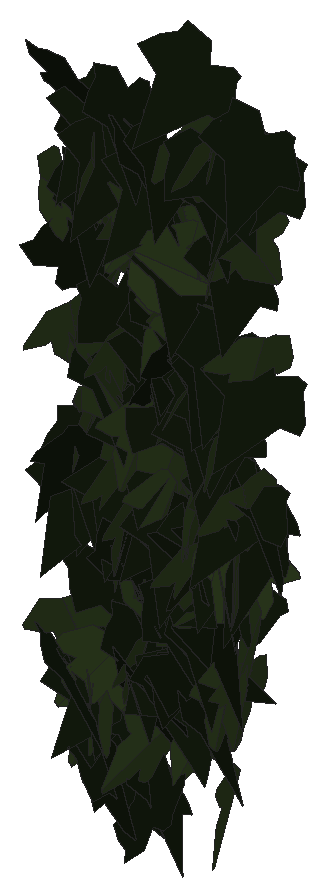
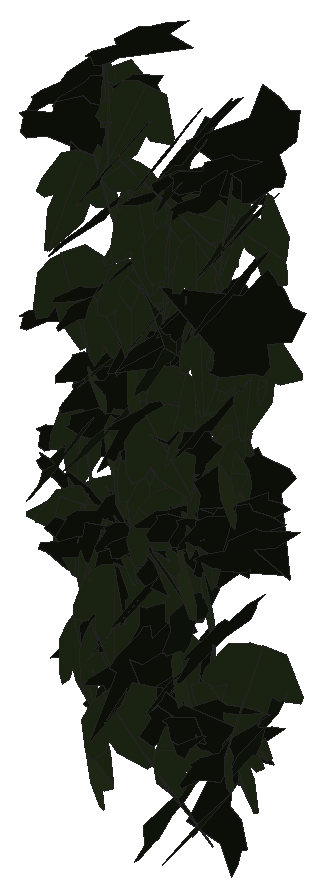
# SketchUp Ruby script. Lengths in inches.
U = 1.inch
M = Sketchup.active_model
def pt(a) = Geom::Point3d.new(a.map { |v| v * U })
def face(e, loops, mat)
  f = e.add_face(loops[0].map { |a| pt(a) })
  loops[1..].each { |l| e.add_face(l.map { |a| pt(a) }).erase! }
  f.material = f.back_material = mat if mat
  f
end
# faces: each face lists its corners as indices into pts; further lists are holes
def faces(e, pts, list, mat = nil) = list.each { |f| face(e, (f[0].is_a?(Array) ? f : [f]).map { |l| l.map { |i| pts[i] } }, mat) }
# xy, xz, yz: faces in a plane at the given z, y or x. An outline is a flat list of corners, or four numbers for a rectangle; further outlines are holes
def ring(l) = l.size == 4 ? [[l[0], l[1]], [l[2], l[1]], [l[2], l[3]], [l[0], l[3]]] : l.each_slice(2).to_a
def flat(e, list, mat, &to3) = list.each { |f| face(e, (f[0].is_a?(Array) ? f : [f]).map { |l| ring(l).map { |u, v| to3.(u, v) } }, mat) }
def xy(e, z, list, mat = nil) = flat(e, list, mat) { |x, y| [x, y, z] }
def xz(e, y, list, mat = nil) = flat(e, list, mat) { |x, z| [x, y, z] }
def yz(e, x, list, mat = nil) = flat(e, list, mat) { |y, z| [x, y, z] }
def lines(e, pts, list) = list.each { |a, b| e.add_line(pt(pts[a]), pt(pts[b])) }
# prism: a flat outline (further loops are holes) pulled along v
def prism(e, loops, v, mat = nil)
  f = face(e, loops, mat); d = Geom::Vector3d.new(v.map { |x| x * U })
  f.pushpull(f.normal.samedirection?(d) ? d.length : -d.length)
end
def box(e, o, s, mat = nil) = prism(e, [[o, [o[0] + s[0], o[1], o[2]], [o[0] + s[0], o[1] + s[1], o[2]], [o[0], o[1] + s[1], o[2]]]], [0, 0, s[2]], mat)
def at(x, y, z, deg = 0) = Geom::Transformation.translation(pt([x, y, z])) * Geom::Transformation.rotation(ORIGIN, Z_AXIS, deg.degrees)
def axes(o, x, y, z) = Geom::Transformation.new([*x, 0, *y, 0, *z, 0, *pt(o).to_a, 1])
def part(name) = M.definitions.add(name)
# library, detail: a bought-in or finely detailed component or shape, given as its bounding box
def library(name, o, s) = part(name).tap { |d| box(d.entities, o, s) }
def detail(e, o, s) = box(e.add_group.entities, o, s)
def put(e, d, t, mat = nil) = e.add_instance(d, t).tap { |i| i.material = mat if mat }
def group(e, t, mat = nil) = e.add_group.tap { |g| g.transformation = t; g.material = mat if mat }.entities
root = M.entities
M.materials.add("efeu1").color = [18, 25, 13]
M.materials.add("efeu2").color = [43, 57, 29]
c1 = part("ivyleaf_9")
p = [[1.54,2.16,1.25],[1.36,2.04,1.19],[-0.21,0.99,0.68],[-0.71,1.11,0.82],[-0.85,0.86,0.67],[-0.8,0.17,0.21],
  [-0.9,-0.01,0.1],[-0.67,-0.16,-0.02],[-0.08,-0.08,-0.05],[-0.03,-0.6,-0.4],[0.65,-0.88,-0.66],[0.83,-0.6,-0.49],
  [1.29,-0.42,-0.43],[1.8125,-0.07,-0.26],[1.21,0.44,0.15]]
faces(c1.entities,p,[[0,1,2,3,4,5,6,7,8,9,10,11,12,13,14]],"efeu1")
c2 = part("ivyleaf_10")
p = [[0,0.5,-0.03],[-0.0625,2.02,-0.43],[-0.19,2.01,-0.46],[-0.54,1.05,-0.29],[-0.52,0.625,-0.18],[-0.83,0.76,-0.28],
  [-1.16,0.64,-0.33],[-1.15,0.33,-0.24],[-0.77,-0.39,0.02],[-0.3,-0.51,0.16],[0.04,-0.48,0.23],[-0.02,2.01,-0.4375],
  [-0.06,2.01,-0.43],[0.04,-0.49,0.23],[0.67,-0.49,0.14],[1.38,0.36,-0.2],[1.375,0.51,-0.24],[0.81,0.65,-0.19],
  [0.62,0.59,-0.15],[0.6,1.09,-0.28],[0.5,1.23,-0.31]]
faces(c2.entities,p,[[0,1,2,3,4,5,6,7,8,9,10],[11,12,0,13,14,15,16,17,18,19,20]],"efeu2")
put(root,c1,axes([22.86,222.96,230.22],[0.08833,-0.4463,-0.20739],[-0.02573,0.20623,-0.45476],[0.49146,0.09101,0.01347]))
put(root,c2,axes([23.15,223.3,223.84],[-0.02881,-0.15896,0.47318],[0.07947,-0.46938,-0.15285],[0.4928,0.0664,0.05231]))
put(root,c2,axes([23.02,223.03,227.23],[0.1477,-0.47388,0.06016],[0.02404,-0.05552,-0.49633],[0.47708,0.14951,0.00638]))
put(root,c2,axes([21.75,222.98,231.33],[-0.01778,-0.00473,0.49966],[0.49964,-0.00651,0.01771],[0.00633,0.49994,0.00496]))
put(root,c1,axes([22.25,223.23,231.43],[0.03847,-0.47216,0.15996],[0.03093,-0.15786,-0.47342],[0.49756,0.04632,0.01706]))
put(root,c2,axes([22.98,222.91,229.69],[-0.00486,-0.49041,-0.09735],[0.00651,0.09728,-0.4904],[0.49993,-0.00603,0.00544]))
put(root,c1,axes([23.97,223.3125,233.67],[-0.30955,-0.34814,0.18161],[-0.04977,-0.1946,-0.45788],[0.38949,-0.30155,0.08582]))
put(root,c2,axes([24.42,223.2,228.96],[0.19071,-0.36763,0.28013],[0.1358,-0.2451,-0.41411],[0.4418,0.23404,0.00636]))
put(root,c2,axes([24.61,223.16,227.08],[-0.16491,0.29275,-0.37027],[0.10502,-0.35963,-0.33112],[-0.46019,-0.18698,0.05713]))
put(root,c1,axes([24.34,223.07,226.03],[-0.15159,-0.00545,-0.47643],[0.47475,0.04065,-0.15152],[0.04038,-0.49832,-0.00715]))
put(root,c2,axes([24.29,222.95,232.79],[0.04442,-0.49195,-0.07754],[0.00767,0.07852,-0.49374],[0.49796,0.04267,0.01452]))
put(root,c1,axes([24.39,223.27,229.91],[-0.11221,-0.47814,0.09379],[-0.00603,-0.09487,-0.49088],[0.48721,-0.11129,0.01552]))
put(root,c2,axes([24.09,223,226.91],[-0.07675,-0.49389,-0.01342],[0.00355,0.01303,-0.49982],[0.49406,-0.07682,0.00151]))
put(root,c1,axes([23.09,222.97,226.24],[-0.12939,-0.06336,0.47879],[0.45684,-0.1769,0.10004],[0.15672,0.46335,0.10367]))
put(root,c1,axes([25.01,223.3125,229.57],[-0.27863,-0.39715,0.12099],[-0.01077,-0.13875,-0.48024],[0.41503,-0.27022,0.06877]))
put(root,c1,axes([23.63,223.29,230.82],[-0.02142,-0.47188,0.16393],[0.03554,-0.16511,-0.47061],[0.49828,-0.00851,0.04061]))
put(root,c2,axes([22.625,222.99,231.35],[-0.32203,0.11672,-0.36424],[0.34419,-0.11924,-0.34251],[-0.16681,-0.47134,-0.00355]))
put(root,c1,axes([22.29,223.03,227.92],[-0.03278,0.36396,-0.34126],[0.02608,-0.34028,-0.36542],[-0.49824,-0.04176,0.00332]))
put(root,c2,axes([23.7,223.25,230.22],[-0.13326,-0.35698,0.32374],[-0.00762,-0.33429,-0.37174],[0.48185,-0.10401,0.08366]))
put(root,c1,axes([21.8,223.17,224.61],[0.2499,-0.3976,0.17165],[0.09149,-0.14523,-0.46961],[0.4233,0.26612,0.00017]))
put(root,c1,axes([23.68,222.56,229.48],[0.11001,0.28622,0.39494],[0.15441,0.3636,-0.30652],[-0.46266,0.18941,-0.0084]))
put(root,c2,axes([22.6875,222.92,228.73],[-0.29006,0.11419,-0.39093],[-0.36407,0.1424,0.31172],[0.18253,0.46549,0.00054]))
put(root,c1,axes([24.75,223.28,227.92],[-0.35549,-0.34847,0.04682],[-0.01764,-0.04882,-0.4973],[0.35116,-0.35522,0.02242]))
put(root,c2,axes([22.44,223.01,224.18],[0.43207,-0.21733,-0.12681],[-0.10618,0.07096,-0.48341],[0.22812,0.44467,0.01517]))
put(root,c2,axes([23.16,223.1875,228.45],[-0.14924,-0.43249,0.2017],[0.01101,-0.2144,-0.45157],[0.47708,-0.13035,0.07352]))
put(root,c2,axes([24.14,223.19,227.875],[0.20825,-0.41714,0.18063],[0.07426,-0.1648,-0.46618],[0.44846,0.22099,-0.00668]))
put(root,c2,axes([24.43,223.08,231.59],[0.27301,-0.41888,0.00251],[-0.00001,-0.003,-0.49999],[0.41889,0.27301,-0.00165]))
put(root,c2,axes([23.625,222.7,231.05],[0.09534,0.23118,0.43298],[0.17159,0.39754,-0.25004],[-0.45986,0.19626,-0.00353]))
put(root,c1,axes([23.35,223.37,231.8125],[-0.27472,-0.37614,0.18179],[-0.05475,-0.18328,-0.46196],[0.41416,-0.27373,0.05952]))
put(root,c1,axes([23.34,223.36,232.21],[0.01894,-0.43265,0.24992],[0.02312,-0.24907,-0.43293],[0.49911,0.02795,0.01057]))
put(root,c2,axes([22.1,222.96,229.67],[-0.17284,-0.45383,-0.11903],[0.05122,0.10784,-0.48554],[0.46637,-0.18004,0.00922]))
put(root,c1,axes([22.61,223.37,232.02],[-0.20321,-0.426,0.165],[-0.04127,-0.16273,-0.47097],[0.45497,-0.20504,0.03097]))
put(root,c1,axes([24.31,223.03,232.8],[-0.04489,-0.38512,-0.3157],[0.06678,0.30946,-0.38701],[0.49348,-0.07691,0.02365]))
put(root,c1,axes([23.59,223.14,226.02],[0.18729,-0.45597,-0.08375],[-0.0255,0.08006,-0.49289],[0.4629,0.1889,0.00673]))
put(root,c1,axes([23.85,222.79,225.46],[0.02851,0.00436,-0.49917],[0.1502,0.47674,0.01274],[0.47605,-0.15068,0.02587]))
put(root,c2,axes([22.46,222.91,231.89],[0.1637,-0.40747,-0.2391],[0.02953,0.26137,-0.42522],[0.47152,0.1251,0.10964]))
put(root,c1,axes([23.23,223.22,224.1],[0.37413,-0.24537,0.22321],[-0.18632,0.12292,0.44741],[-0.27444,-0.41795,0.00055]))
put(root,c1,axes([24.09,223.46,229.13],[-0.12274,-0.37882,0.30237],[0.08857,-0.32419,-0.37021],[0.47654,-0.03732,0.14668]))
put(root,c2,axes([24.92,223.18,230],[-0.19279,-0.45191,0.09277],[-0.01999,-0.09227,-0.49101],[0.4609,-0.19303,0.01751]))
put(root,c2,axes([24.78,223.03,227.96],[-0.12237,-0.46835,-0.12521],[0.04271,0.11822,-0.48394],[0.48291,-0.12914,0.01107]))
put(root,c1,axes([24.79,223.42,232.89],[-0.14424,-0.46381,0.11865],[-0.00796,-0.12157,-0.48493],[0.47868,-0.14178,0.02769]))
put(root,c2,axes([23.84,223.4,227.64],[0.0936,-0.27919,0.40409],[0.24151,-0.33204,-0.28535],[0.42768,0.2486,0.0727]))
put(root,c1,axes([23.18,223.43,229.44],[0.0297,-0.38591,0.31652],[0.10535,-0.30509,-0.38186],[0.48787,0.08938,0.06319]))
put(root,c2,axes([22.5,223.14,224.82],[0.41456,-0.01294,-0.27923],[-0.27895,0.01299,-0.41475],[0.01799,0.49966,0.00355]))
put(root,c1,axes([22.93,223.23,232.32],[0.27368,-0.41416,0.05971],[0.02588,-0.05446,-0.49635],[0.41765,0.27478,-0.00837]))
put(root,c1,axes([21.65,223.13,232.85],[0.34092,-0.17815,0.31943],[0.28597,-0.14241,-0.38463],[0.22803,0.44495,0.00479]))
put(root,c1,axes([23.5,222.83,222.9375],[-0.41726,0.18998,-0.19952],[-0.18595,0.07297,0.45836],[0.20328,0.45671,0.00975]))
put(root,c1,axes([22.14,223.43,227.125],[-0.27659,-0.40638,0.09142],[-0.02251,-0.09499,-0.49038],[0.41592,-0.27538,0.03425]))
put(root,c2,axes([22.98,223.17,226.13],[0.12027,-0.08451,-0.4779],[0.45878,-0.14078,0.14035],[-0.15828,-0.47227,0.04368]))
put(root,c1,axes([24.4,223.45,231],[-0.06149,-0.46571,0.17127],[0.05266,-0.17773,-0.46437],[0.4934,-0.03907,0.0709]))
put(root,c2,axes([24.32,223.32,225.09],[0.01246,-0.44884,0.21997],[0.1506,-0.20644,-0.42977],[0.47662,0.07696,0.13005]))
put(root,c1,axes([24.18,223.33,228.78],[-0.17737,-0.46356,-0.06046],[0.00638,0.06226,-0.49607],[0.46744,-0.17675,-0.01617]))
put(root,c1,axes([22.6875,223.35,232.84],[0.08267,-0.49019,0.05362],[0.00269,-0.05392,-0.49708],[0.49311,0.08248,-0.00628]))
put(root,c2,axes([22.02,223.06,225.36],[-0.43186,-0.22409,-0.11524],[0.10209,0.05347,-0.48654],[0.23038,-0.44376,-0.00043]))
put(root,c1,axes([23.86,223.42,225.55],[0.09728,-0.45755,0.17658],[0.04698,-0.1705,-0.46768],[0.48819,0.10758,0.00982]))
put(root,c1,axes([22.28,223.26,223.33],[-0.0292,-0.02934,-0.49828],[0.49591,0.05501,-0.0323],[0.05672,-0.4961,0.02589]))
put(root,c2,axes([23.41,223.34,227.47],[-0.08875,-0.45001,0.19903],[0.02537,-0.20616,-0.45481],[0.49141,-0.07063,0.05943]))
put(root,c1,axes([22.71,223.42,225.95],[0.13874,-0.29865,0.37625],[0.18108,-0.33022,-0.32888],[0.44493,0.22752,0.01653]))
put(root,c1,axes([23.87,223.31,224.58],[0.27044,-0.40584,0.11026],[0.06109,-0.09179,-0.48769],[0.41609,0.27725,-0.00006]))
put(root,c2,axes([24.28,223.42,223.43],[0.18264,-0.31008,0.34713],[0.21577,-0.274,-0.35828],[0.41241,0.28067,0.03372]))
put(root,c2,axes([23.02,223.22,225.13],[0.14598,-0.47818,-0.00606],[-0.00186,0.00577,-0.49996],[0.47821,0.14599,-0.00009]))
put(root,c2,axes([24.84,223.14,226.11],[0.32424,-0.34674,-0.15698],[-0.08491,0.13513,-0.47385],[0.37103,0.33393,0.02874]))
put(root,c1,axes([23.5625,222.875,229.64],[-0.36594,0.17779,-0.29065],[-0.26069,0.12854,0.40684],[0.21939,0.4493,-0.00137]))
put(root,c2,axes([23.72,223.22,231.71],[-0.4711,0.08902,-0.14193],[0.11316,-0.14325,-0.46548],[-0.12354,-0.4707,0.11482]))
put(root,c1,axes([23.21,223.32,230.25],[0.2049,-0.45596,-0.01072],[-0.00472,0.00963,-0.49988],[0.45606,0.20495,-0.00036]))
put(root,c2,axes([22.44,222.86,229.6],[0.10239,-0.16983,0.45899],[-0.21694,0.40459,0.19809],[-0.43869,-0.23971,0.00917]))
put(root,c1,axes([22.87,223.43,225.16],[0.09465,-0.48331,0.08635],[0.00192,-0.08757,-0.49227],[0.49096,0.09352,-0.01472]))
put(root,c1,axes([23.29,223.48,229.8125],[-0.02095,-0.49022,0.09613],[-0.00265,-0.0961,-0.49067],[0.49955,-0.02107,0.00143]))
put(root,c1,axes([22.6,223.46,224.57],[-0.40176,-0.28961,0.06868],[-0.0588,-0.03587,-0.49523],[0.29177,-0.40601,-0.00523]))
put(root,c1,axes([24.76,223.39,227.24],[-0.40868,-0.12862,-0.25776],[0.26854,-0.00819,-0.42169],[0.10425,-0.48311,0.07577]))
put(root,c1,axes([24.01,223.05,226.78],[-0.32309,0.32998,0.19164],[-0.13,0.1409,-0.46179],[-0.35876,-0.34822,-0.00525]))
put(root,c2,axes([23.45,223.26,227.88],[-0.37147,-0.28989,0.16726],[-0.12582,-0.11059,-0.4711],[0.31013,-0.39209,0.00922]))
put(root,c1,axes([23.14,223.29,227.03],[-0.01515,-0.15061,-0.47654],[0.46333,0.17448,-0.06988],[0.18734,-0.4437,0.13428]))
put(root,c1,axes([22.4375,223.51,232.46],[-0.3517,-0.35069,0.05763],[-0.01055,-0.07074,-0.49486],[0.35524,-0.3493,0.04236]))
put(root,c1,axes([23.5625,223.47,227.0625],[-0.18733,-0.46355,-0.00522],[0.00312,0.00437,-0.49997],[0.46357,-0.18735,0.00125]))
put(root,c1,axes([22.36,223.43,228.97],[0.09049,-0.49081,0.03032],[0.00874,-0.02922,-0.49907],[0.49167,0.09085,0.00329]))
put(root,c2,axes([22.75,223.18,226.4375],[0.27011,-0.39053,-0.15662],[-0.06817,0.14304,-0.47423],[0.4152,0.27754,0.02402]))
put(root,c1,axes([23.6,223.33,224.92],[-0.10456,-0.43771,-0.21789],[0.1155,0.1944,-0.44595],[0.47511,-0.14359,0.06046]))
put(root,c2,axes([24.32,223.23,226.61],[-0.22485,0.42948,-0.12241],[0.05471,-0.10952,-0.48478],[-0.44322,-0.2314,0.00226]))
put(root,c2,axes([22.96,223.45,231.3],[-0.31777,-0.26522,0.2805],[-0.08677,-0.30494,-0.38663],[0.37616,-0.2944,0.14777]))
put(root,c2,axes([22.83,223.35,226.16],[0.28926,-0.35996,-0.19173],[0.11391,-0.1544,0.46172],[-0.3916,-0.31079,-0.00731]))
put(root,c1,axes([23.92,223.45,232.1],[0.13375,-0.47837,0.05722],[0.01381,-0.05555,-0.49671],[0.48158,0.13445,-0.00165]))
put(root,c2,axes([24.12,223.23,225.86],[-0.26533,-0.42301,-0.02572],[0.01286,0.02229,-0.49934],[0.4236,-0.26564,-0.00095]))
put(root,c1,axes([24.11,223.43,229.2],[-0.20405,-0.43745,-0.13039],[0.05491,0.11826,-0.4827],[0.45315,-0.21131,-0.00023]))
put(root,c2,axes([22.06,223.52,228.28],[0.15503,-0.35638,0.31458],[0.16147,-0.27173,-0.38742],[0.44709,0.22171,0.03083]))
put(root,c2,axes([23.875,223.07,232.74],[-0.17505,-0.36493,-0.29356],[0.13743,0.25958,-0.40464],[0.44774,-0.22236,0.00942]))
put(root,c2,axes([24.5,223.33,227.05],[0.33227,0.35434,-0.11847],[-0.06871,-0.09788,-0.48549],[-0.36725,0.33891,-0.01635]))
put(root,c1,axes([22.33,223.19,223.49],[0.32169,-0.33269,-0.1893],[-0.06775,0.19388,-0.45587],[0.37673,0.31895,0.07966]))
put(root,c2,axes([23.72,223.23,228.95],[0.10756,-0.46777,-0.14007],[-0.03703,0.1352,-0.47995],[0.48689,0.11362,-0.00556]))
put(root,c1,axes([23.0625,223.47,228.35],[-0.30099,-0.36379,-0.16451],[0.11307,0.11991,-0.47206],[0.38291,-0.32137,0.01009]))
put(root,c1,axes([24.8,223.55,232.48],[-0.38,-0.32496,0.00206],[-0.00156,-0.00135,-0.5],[0.32496,-0.38,0.00001]))
put(root,c2,axes([22.59,223.34,227.52],[0.02783,-0.4985,-0.02689],[0.00699,0.02732,-0.4992],[0.49918,0.02741,0.00849]))
put(root,c1,axes([22.13,223.59,224.31],[-0.11154,-0.48616,0.03478],[-0.00775,-0.0339,-0.49879],[0.48734,-0.11181,0.00003]))
put(root,c1,axes([22.65,223.53,227.41],[-0.30921,-0.37617,-0.11352],[0.07565,0.08477,-0.48692],[0.38558,-0.31829,0.00449]))
put(root,c2,axes([24.23,223.23,232.95],[0.23363,-0.39223,-0.20388],[-0.03398,0.21399,-0.45061],[0.44075,0.22441,0.07334]))
put(root,c2,axes([24.51,223.45,225.11],[0.01404,-0.49107,0.093],[0.06531,-0.09044,-0.4874],[0.49552,0.02583,0.06161]))
put(root,c1,axes([23.97,223.59,228.24],[0.08404,-0.47458,0.13307],[0.09071,-0.11779,-0.47739],[0.48447,0.10438,0.06631]))
put(root,c2,axes([23.89,223.55,224.29],[-0.23063,-0.35787,0.26218],[-0.04239,-0.27637,-0.41452],[0.4416,-0.21343,0.09714]))
put(root,c2,axes([23.77,223.3,230.36],[-0.17161,-0.46314,-0.07778],[0.01589,0.07704,-0.49377],[0.46936,-0.17194,-0.01172]))
put(root,c1,axes([24.68,223.54,226.41],[-0.42493,-0.07609,0.25228],[-0.24853,-0.04334,-0.43169],[0.08756,-0.49227,-0.00098]))
put(root,c2,axes([23.18,223.18,231.08],[0.11725,-0.40209,-0.27309],[-0.00576,0.27976,-0.41437],[0.48602,0.10032,0.06097]))
put(root,c1,axes([23.53,223.15,231.61],[-0.15539,0.31505,0.3558],[-0.30262,0.22304,-0.32966],[-0.36644,-0.3178,0.12136]))
put(root,c2,axes([22.72,223.33,231.1],[-0.02811,-0.49095,-0.09045],[0.02204,0.08928,-0.49147],[0.49872,-0.03162,0.01662]))
put(root,c1,axes([22.95,223.58,223.13],[0.18967,-0.44009,0.14263],[0.05982,-0.12953,-0.47921],[0.45874,0.19885,0.00352]))
put(root,c2,axes([24.71,223.21,231.52],[-0.17596,-0.39689,-0.24802],[0.11244,0.22136,-0.434],[0.45431,-0.20851,0.01135]))
put(root,c1,axes([21.78,223.2,230.14],[0.07606,-0.05717,0.49086],[0.49134,0.06192,-0.06893],[-0.05291,0.49285,0.0656]))
put(root,c2,axes([22.53,223.16,228.03],[-0.14202,0.13361,-0.46041],[-0.34047,0.30994,0.19497],[0.3375,0.36889,0.00294]))
put(root,c1,axes([24.05,223.62,227.11],[-0.1992,-0.4584,-0.01366],[0.005,0.01272,-0.49981],[0.45858,-0.19926,-0.00048]))
put(root,c2,axes([23.2,223.68,227.32],[-0.11843,-0.33656,0.35028],[0.13153,-0.36929,-0.31036],[0.46762,0.01863,0.17601]))
put(root,c1,axes([23.34,223.74,227.1],[-0.2585,-0.37657,0.20341],[-0.06717,-0.19899,-0.45375],[0.42269,-0.26192,0.05229]))
put(root,c2,axes([23.52,223.4375,231.4],[-0.13037,-0.48208,0.02451],[-0.00455,-0.02416,-0.4994],[0.48268,-0.13044,0.00191]))
put(root,c1,axes([24.62,223.63,227.7],[0.14601,-0.45457,0.14848],[0.05191,-0.13926,-0.4774],[0.47538,0.15482,0.00653]))
put(root,c1,axes([23.6,223.19,225.1875],[0.16438,-0.23761,-0.40807],[-0.19597,0.3588,-0.28786],[0.42962,0.25457,0.02483]))
put(root,c1,axes([22.06,223.58,227.68],[-0.11198,-0.47844,-0.0925],[0.01848,0.09067,-0.49136],[0.48695,-0.11346,-0.00262]))
put(root,c1,axes([22.25,223.62,227.57],[-0.29932,-0.39486,-0.06701],[0.03058,0.06088,-0.49534],[0.39934,-0.30063,-0.01229]))
put(root,c1,axes([23,223.29,224.33],[-0.43414,-0.04321,-0.24424],[-0.243,-0.02458,0.43629],[-0.04971,0.49752,0.00035]))
put(root,c1,axes([21.9,223.72,231.79],[0.06317,-0.439,0.23084],[0.05552,-0.22498,-0.44306],[0.49288,0.08161,0.02032]))
put(root,c1,axes([22.14,223.76,224.2],[-0.02777,-0.43013,0.25342],[0.04016,-0.25491,-0.42826],[0.49761,-0.00343,0.0487]))
put(root,c1,axes([21.95,223.7,230.97],[0.04569,-0.47426,0.15162],[0.00075,-0.15219,-0.47627],[0.49791,0.04375,-0.01319]))
put(root,c2,axes([23.05,223.32,229.05],[-0.45394,0.20381,0.04896],[-0.04558,0.01801,-0.49759],[-0.20459,-0.45622,0.00223]))
put(root,c2,axes([24.5,223.41,226.79],[0.4312,0.23976,0.08116],[0.07452,0.03295,-0.49332],[-0.2419,0.43753,-0.00732]))
put(root,c2,axes([21.88,223.72,224.45],[-0.01373,-0.10896,0.48779],[0.36015,-0.34051,-0.06593],[0.34656,0.34954,0.08783]))
put(root,c1,axes([22.19,223.4,226.05],[0.21447,-0.39708,-0.21524],[-0.03868,0.22125,-0.44671],[0.45001,0.20826,0.06418]))
put(root,c2,axes([23.15,223.63,228.53],[-0.20437,-0.39406,0.2301],[-0.03797,-0.23657,-0.43885],[0.45474,-0.19685,0.06677]))
put(root,c2,axes([23.94,223.66,230.01],[-0.00027,-0.44129,0.23509],[0.06079,-0.23337,-0.438],[0.49629,0.02835,0.05378]))
put(root,c1,axes([23.22,223.39,228.75],[0.12873,-0.38577,-0.29088],[0.05477,0.31074,-0.38787],[0.48003,0.068,0.12226]))
